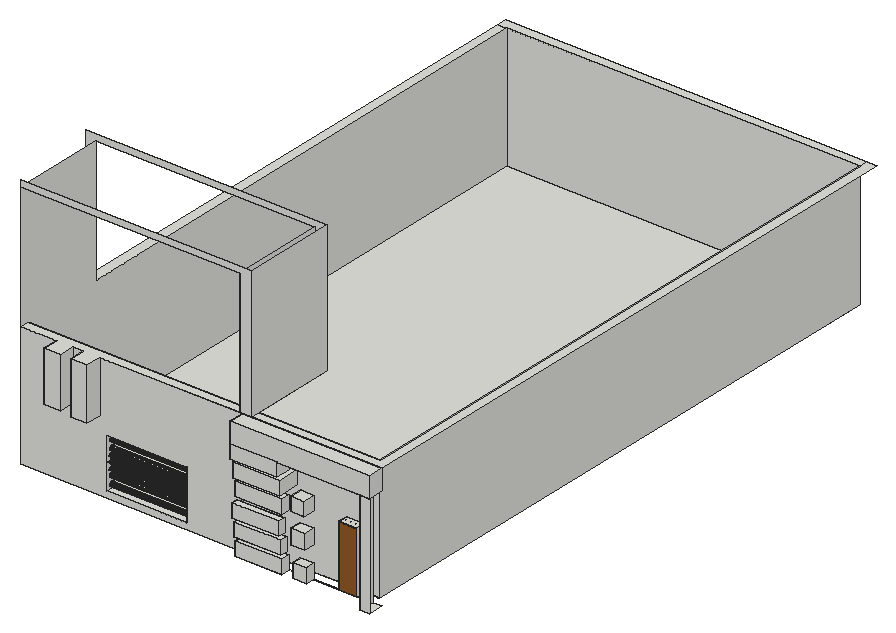
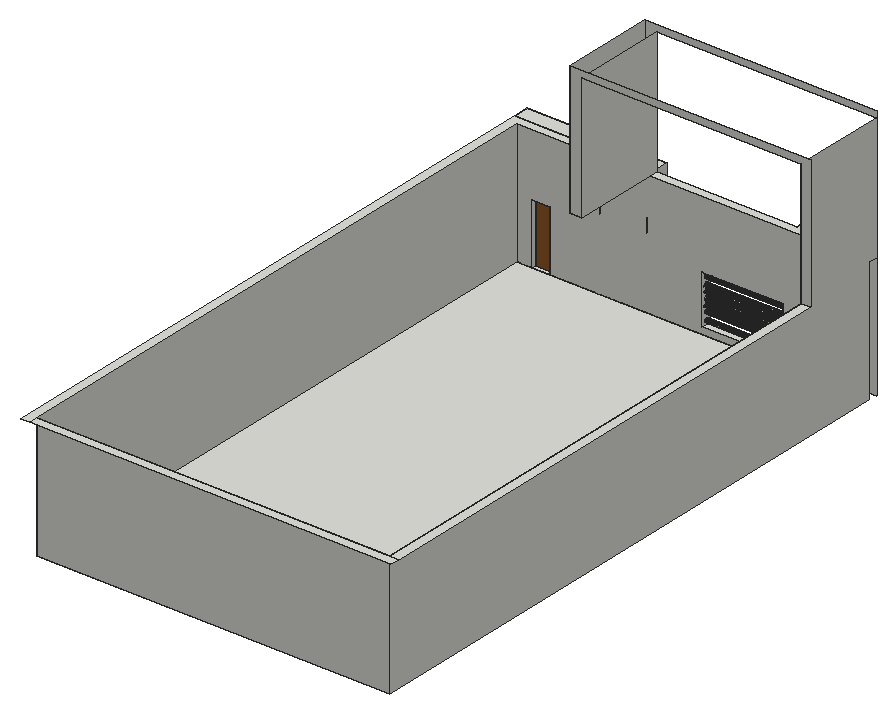
# SketchUp Ruby script. Lengths in inches.
U = 1.inch
M = Sketchup.active_model
def pt(a) = Geom::Point3d.new(a.map { |v| v * U })
def face(e, loops, mat)
  f = e.add_face(loops[0].map { |a| pt(a) })
  loops[1..].each { |l| e.add_face(l.map { |a| pt(a) }).erase! }
  f.material = f.back_material = mat if mat
  f
end
# faces: each face lists its corners as indices into pts; further lists are holes
def faces(e, pts, list, mat = nil) = list.each { |f| face(e, (f[0].is_a?(Array) ? f : [f]).map { |l| l.map { |i| pts[i] } }, mat) }
# xy, xz, yz: faces in a plane at the given z, y or x. An outline is a flat list of corners, or four numbers for a rectangle; further outlines are holes
def ring(l) = l.size == 4 ? [[l[0], l[1]], [l[2], l[1]], [l[2], l[3]], [l[0], l[3]]] : l.each_slice(2).to_a
def flat(e, list, mat, &to3) = list.each { |f| face(e, (f[0].is_a?(Array) ? f : [f]).map { |l| ring(l).map { |u, v| to3.(u, v) } }, mat) }
def xy(e, z, list, mat = nil) = flat(e, list, mat) { |x, y| [x, y, z] }
def xz(e, y, list, mat = nil) = flat(e, list, mat) { |x, z| [x, y, z] }
def yz(e, x, list, mat = nil) = flat(e, list, mat) { |y, z| [x, y, z] }
def lines(e, pts, list) = list.each { |a, b| e.add_line(pt(pts[a]), pt(pts[b])) }
# prism: a flat outline (further loops are holes) pulled along v
def prism(e, loops, v, mat = nil)
  f = face(e, loops, mat); d = Geom::Vector3d.new(v.map { |x| x * U })
  f.pushpull(f.normal.samedirection?(d) ? d.length : -d.length)
end
def box(e, o, s, mat = nil) = prism(e, [[o, [o[0] + s[0], o[1], o[2]], [o[0] + s[0], o[1] + s[1], o[2]], [o[0], o[1] + s[1], o[2]]]], [0, 0, s[2]], mat)
def at(x, y, z, deg = 0) = Geom::Transformation.translation(pt([x, y, z])) * Geom::Transformation.rotation(ORIGIN, Z_AXIS, deg.degrees)
def axes(o, x, y, z) = Geom::Transformation.new([*x, 0, *y, 0, *z, 0, *pt(o).to_a, 1])
def part(name) = M.definitions.add(name)
# library, detail: a bought-in or finely detailed component or shape, given as its bounding box
def library(name, o, s) = part(name).tap { |d| box(d.entities, o, s) }
def detail(e, o, s) = box(e.add_group.entities, o, s)
def put(e, d, t, mat = nil) = e.add_instance(d, t).tap { |i| i.material = mat if mat }
def group(e, t, mat = nil) = e.add_group.tap { |g| g.transformation = t; g.material = mat if mat }.entities
root = M.entities
M.materials.add("[Wood Floor Parquet]").color = [145, 89, 39]
c1 = part("ZZZ")
g1 = group(c1.entities,at(61.03,0,0))
box(g1,[-61.03,0,0],[61.03,1.5625,79.28])
box(root,[224.5625,43.74,143.55],[45.75,6.75,13.12])
box(root,[224.5625,41.22,160.97],[45.75,6.32,13.13])
xy(root,126,[[9.02,62.875,351,644.4375]])
xy(root,126.125,[[351,38.75,360,53.4375],[224.5625,44.875,224.5625,53.875,318.32,53.875,318.32,53.4375,270.3125,53.4375,270.3125,44.875],[335.64,53.4375,351,53.875],[318.32,53.875,335.64,62.875]])
xy(root,127.16,[[281.07,44.125,294.45,53.4375]])
xy(root,132.42,[[92.77,53.875,170.95,62.875]])
xy(root,139.25,[[224.5625,44.875,270.3125,53.4375]])
xy(root,140.53,[[281.07,44.125,294.45,53.4375]])
xy(root,156.97,[[280.4375,42.25,294.5,53.4375]])
xy(root,171.03,[[280.4375,42.25,294.5,53.4375]])
xy(root,178.4,[[224.5625,44.59,270.3125,53.4375]])
xy(root,180.73,[[92.77,53.875,170.95,62.875]])
xy(root,185.5,[[318.32,53.4375,335.64,62.875]])
xy(root,186.3,[[281.15,41.8125,294.21,53.4375]])
xy(root,191.52,[[224.5625,44.59,270.3125,53.4375]])
xy(root,195.5625,[[70.08,38.75,85.7,53.875]])
xy(root,195.82,[[224.5625,41.64,270.3125,62.57]])
xy(root,197.1875,[[43.99,38.75,60.12,53.875]])
xy(root,199.36,[[281.15,41.8125,294.21,53.4375]])
xy(root,208.95,[[224.5625,41.64,270.3125,62.57]])
xy(root,213.25,[[224.5625,38.6875,270.3125,53.4375]])
xy(root,226.37,[[224.5625,38.6875,270.3125,53.4375],[270.3125,38.6875,270.3125,53.4375,351,53.4375,351,38.75,360,38.75,360,38.6875],[351,38.75,360,53.4375]])
xy(root,246,[[224.5625,38.6875,360,53.875],[43.99,38.75,60.12,38.75,60.12,53.875,70.08,53.875,70.08,38.75,85.7,38.75,85.7,53.875,221.54,53.875,221.54,62.875,9.02,62.875,9.02,53.875,43.99,53.875],[221.54,53.875,233.71,62.875],[233.71,53.875,360,53.875,360,653.4375,351,653.4375,351,62.875,233.71,62.875],[221.54,62.875,233.71,144.86],
  [0,144.86,9.02,644.4375],[0,644.4375,351,653.4375]])
xz(root,38.6875,[[224.5625,213.25,270.3125,226.37],[224.5625,226.37,360,246]])
xz(root,38.75,[[351,126.125,360,226.37],[70.08,195.5625,85.7,246],[43.99,197.1875,60.12,246]])
xz(root,41.64,[[224.5625,195.82,270.3125,208.95]])
xz(root,41.8125,[[281.15,186.3,294.21,199.36]])
xz(root,42.25,[[280.4375,156.97,294.5,171.03]])
xz(root,44.125,[[281.07,127.16,294.45,140.53]])
xz(root,44.59,[[224.5625,178.4,270.3125,191.52]])
xz(root,44.875,[[224.5625,126.125,270.3125,139.25]])
xz(root,53.875,[[[9.02,126.125,224.5625,126.125,224.5625,246,85.7,246,85.7,195.5625,70.08,195.5625,70.08,246,60.12,246,60.12,197.1875,43.99,197.1875,43.99,246,9.02,246],[92.77,132.42,170.95,180.73]],[221.54,246,233.71,246,233.71,373.61,9.02,373.61,9.02,367.15,221.54,367.15]])
xz(root,62.57,[[224.5625,195.82,270.3125,208.95]])
xz(root,62.875,[[9.02,126,351,126.125],[[9.02,126.125,9.02,246,351,246,351,126.125,335.64,126.125,335.64,185.5,318.32,185.5,318.32,126.125],[92.77,132.42,170.95,180.73]]])
xz(root,144.86,[[0,246,0,373.61,233.71,373.61,233.71,246,221.54,246,221.54,367.15,9.02,367.15,9.02,246]])
xz(root,644.4375,[[9.02,126,351,246]])
yz(root,9.02,[[62.875,126,644.4375,126,644.4375,246,144.86,246,144.86,367.15,53.875,367.15,53.875,246,62.875,246]])
yz(root,43.99,[[38.75,197.1875,53.875,246]])
yz(root,60.12,[[38.75,197.1875,53.875,246]])
yz(root,70.08,[[38.75,195.5625,53.875,246]])
yz(root,85.7,[[38.75,195.5625,53.875,246]])
yz(root,92.77,[[53.875,132.42,62.875,180.73]])
yz(root,170.95,[[53.875,132.42,62.875,180.73]])
yz(root,221.54,[[53.875,246,144.86,367.15]])
yz(root,224.5625,[[44.875,126.125,44.875,139.25,53.4375,139.25,53.4375,195.82,53.875,195.82,53.875,126.125],[44.59,178.4,53.4375,191.52],[41.64,195.82,53.4375,208.95],[53.4375,195.82,53.875,208.95],[53.875,195.82,62.57,208.95],
  [53.4375,208.95,53.4375,213.25,38.6875,213.25,38.6875,246,53.875,246,53.875,208.95]])
yz(root,233.71,[[53.875,246,144.86,373.61]])
yz(root,270.3125,[[44.875,126.125,53.4375,139.25],[44.59,178.4,53.4375,191.52],[41.64,195.82,62.57,208.95],[38.6875,213.25,53.4375,226.37]])
yz(root,280.4375,[[42.25,156.97,53.4375,171.03]])
yz(root,281.07,[[44.125,127.16,53.4375,140.53]])
yz(root,281.15,[[41.8125,186.3,53.4375,199.36]])
yz(root,294.21,[[41.8125,186.3,53.4375,199.36]])
yz(root,294.45,[[44.125,127.16,53.4375,140.53]])
yz(root,294.5,[[42.25,156.97,53.4375,171.03]])
yz(root,318.32,[[53.4375,126.125,62.875,185.5]])
yz(root,335.64,[[53.4375,126.125,62.875,185.5]])
yz(root,351,[[62.875,126,644.4375,246],[38.75,126.125,53.4375,226.37]])
yz(root,360,[[38.6875,226.37,53.4375,226.37,53.875,246,38.6875,246]])
p = [[92.77,57.95,135.08],[92.77,58.46,134.97],[171.52,58.46,134.97],[171.52,57.95,135.08],[92.77,58.98,135],[171.52,58.98,135],
  [92.77,59.48,135.16],[171.52,59.48,135.16],[92.77,57.48,135.3125],[171.52,57.48,135.3125],[92.77,59.91,135.45],[171.52,59.91,135.45],
  [92.77,57.09,135.66],[171.52,57.09,135.66],[92.77,60.26,135.84],[171.52,60.26,135.84],[92.77,56.81,136.1],[171.52,56.81,136.1],
  [92.77,60.5,136.3],[171.52,60.5,136.3],[92.77,56.65,136.59],[171.52,56.65,136.59],[92.77,60.61,136.8125],[171.52,60.61,136.8125],
  [92.77,56.62,137.11],[171.52,56.62,137.11],[92.77,60.58,137.33],[171.52,60.58,137.33],[92.77,56.72,137.625],[171.52,56.72,137.625],
  [92.77,60.41,137.83],[171.52,60.41,137.83],[92.77,56.96,138.09],[171.52,56.96,138.09],[92.77,60.13,138.27],[171.52,60.13,138.27],
  [92.77,57.31,138.48],[171.52,57.31,138.48],[92.77,59.74,138.61],[171.52,59.74,138.61],[92.77,57.74,138.77],[171.52,57.74,138.77],
  [92.77,59.27,138.85],[171.52,59.27,138.85],[92.77,58.24,138.93],[171.52,58.24,138.93],[92.77,58.76,138.96],[171.52,58.76,138.96],
  [92.77,57.79,142.92],[92.77,58.3,142.82],[171.52,58.3,142.82],[171.52,57.79,142.92],[92.77,58.82,142.85],[171.52,58.82,142.85],
  [92.77,59.31,143.01],[171.52,59.31,143.01],[92.77,57.32,143.16],[171.52,57.32,143.16],[92.77,59.75,143.3],[171.52,59.75,143.3],
  [92.77,56.93,143.51],[171.52,56.93,143.51],[92.77,60.1,143.68],[171.52,60.1,143.68],[92.77,56.65,143.95],[171.52,56.65,143.95],
  [92.77,60.34,144.15],[171.52,60.34,144.15],[92.77,56.48,144.44],[171.52,56.48,144.44],[92.77,60.44,144.66],[171.52,60.44,144.66],
  [92.77,56.45,144.96],[171.52,56.45,144.96],[92.77,60.41,145.18],[171.52,60.41,145.18],[92.77,56.5625,145.47],[171.52,56.5625,145.47],
  [92.77,60.25,145.68],[171.52,60.25,145.68],[92.77,56.8,145.94],[171.52,56.8,145.94],[92.77,59.96,146.12],[171.52,59.96,146.12],
  [92.77,57.14,146.33],[171.52,57.14,146.33],[92.77,59.58,146.46],[171.52,59.58,146.46],[92.77,57.58,146.61],[171.52,57.58,146.61],
  [92.77,59.11,146.7],[171.52,59.11,146.7],[92.77,58.08,146.78],[171.52,58.08,146.78],[92.77,58.6,146.81],[171.52,58.6,146.81],
  [92.77,57.95,148.64],[92.77,58.46,148.53],[171.52,58.46,148.53],[171.52,57.95,148.64],[92.77,58.98,148.56],[171.52,58.98,148.56],
  [92.77,57.48,148.875],[171.52,57.48,148.875],[92.77,59.48,148.72],[171.52,59.48,148.72],[92.77,59.91,149.01],[171.52,59.91,149.01],
  [92.77,57.09,149.22],[171.52,57.09,149.22],[92.77,60.26,149.4],[171.52,60.26,149.4],[92.77,56.81,149.66],[171.52,56.81,149.66],
  [92.77,60.5,149.86],[171.52,60.5,149.86],[92.77,56.65,150.15],[171.52,56.65,150.15],[92.77,60.61,150.375],[171.52,60.61,150.375],
  [92.77,56.62,150.68],[171.52,56.62,150.68],[92.77,60.58,150.9],[171.52,60.58,150.9],[92.77,56.72,151.1875],[171.52,56.72,151.1875],
  [92.77,60.41,151.39],[171.52,60.41,151.39],[92.77,56.96,151.65],[171.52,56.96,151.65],[92.77,60.13,151.83],[171.52,60.13,151.83],
  [92.77,57.31,152.04],[171.52,57.31,152.04],[92.77,59.74,152.18],[171.52,59.74,152.18],[92.77,57.74,152.33],[171.52,57.74,152.33],
  [92.77,59.27,152.41],[171.52,59.27,152.41],[92.77,58.24,152.49],[171.52,58.24,152.49],[92.77,58.76,152.52],[171.52,58.76,152.52],
  [91.06,58.11,154.6],[91.06,58.625,154.5],[169.81,58.625,154.5],[169.81,58.11,154.6],[91.06,59.15,154.53],[169.81,59.15,154.53],
  [91.06,59.64,154.69],[169.81,59.64,154.69],[91.06,57.65,154.84],[169.81,57.65,154.84],[91.06,60.08,154.98],[169.81,60.08,154.98],
  [91.06,57.26,155.1875],[169.81,57.26,155.1875],[91.06,60.43,155.36],[169.81,60.43,155.36],[91.06,56.97,155.625],[169.81,56.97,155.625],
  [91.06,60.66,155.83],[169.81,60.66,155.83],[91.06,56.81,156.12],[169.81,56.81,156.12],[91.06,60.77,156.34],[169.81,60.77,156.34],
  [91.06,56.78,156.64],[169.81,56.78,156.64],[91.06,60.74,156.86],[169.81,60.74,156.86],[91.06,56.89,157.15],[169.81,56.89,157.15],
  [91.06,60.58,157.36],[169.81,60.58,157.36],[91.06,57.125,157.62],[169.81,57.125,157.62],[91.06,60.29,157.8],[169.81,60.29,157.8],
  [91.06,57.47,158.01],[169.81,57.47,158.01],[91.06,59.9,158.14],[169.81,59.9,158.14],[91.06,57.91,158.29],[169.81,57.91,158.29],
  [91.06,59.4375,158.38],[169.81,59.4375,158.38],[91.06,58.4,158.46],[169.81,58.4,158.46],[91.06,58.93,158.49],[169.81,58.93,158.49],
  [92.77,57.95,160.7],[92.77,58.46,160.59],[171.52,58.46,160.59],[171.52,57.95,160.7],[92.77,58.98,160.62],[171.52,58.98,160.62],
  [92.77,59.48,160.79],[171.52,59.48,160.79],[92.77,57.48,160.9375],[171.52,57.48,160.9375],[92.77,59.91,161.07],[171.52,59.91,161.07],
  [92.77,57.09,161.28],[171.52,57.09,161.28],[92.77,60.26,161.46],[171.52,60.26,161.46],[92.77,56.81,161.72],[171.52,56.81,161.72],
  [92.77,60.5,161.93],[171.52,60.5,161.93],[92.77,56.65,162.22],[171.52,56.65,162.22],[92.77,60.61,162.4375],[171.52,60.61,162.4375],
  [92.77,56.62,162.74],[171.52,56.62,162.74],[92.77,60.58,162.96],[171.52,60.58,162.96],[92.77,56.72,163.25],[171.52,56.72,163.25],
  [92.77,60.41,163.45],[171.52,60.41,163.45],[92.77,56.96,163.72],[171.52,56.96,163.72],[92.77,60.13,163.89],[171.52,60.13,163.89],
  [92.77,57.31,164.1],[171.52,57.31,164.1],[92.77,59.74,164.24],[171.52,59.74,164.24],[92.77,57.74,164.39],[171.52,57.74,164.39],
  [92.77,59.27,164.48],[171.52,59.27,164.48],[92.77,58.24,164.55],[171.52,58.24,164.55],[92.77,58.76,164.58],[171.52,58.76,164.58],
  [92.77,57.95,166.14],[92.77,58.46,166.03],[171.52,58.46,166.03],[171.52,57.95,166.14],[92.77,58.98,166.06],[171.52,58.98,166.06],
  [92.77,57.48,166.375],[171.52,57.48,166.375],[92.77,59.48,166.22],[171.52,59.48,166.22],[92.77,59.91,166.51],[171.52,59.91,166.51],
  [92.77,57.09,166.72],[171.52,57.09,166.72],[92.77,60.26,166.9],[171.52,60.26,166.9],[92.77,56.81,167.16],[171.52,56.81,167.16],
  [92.77,60.5,167.36],[171.52,60.5,167.36],[92.77,56.65,167.65],[171.52,56.65,167.65],[92.77,60.61,167.875],[171.52,60.61,167.875],
  [92.77,56.62,168.18],[171.52,56.62,168.18],[92.77,60.58,168.4],[171.52,60.58,168.4],[92.77,56.72,168.6875],[171.52,56.72,168.6875],
  [92.77,60.41,168.89],[171.52,60.41,168.89],[92.77,56.96,169.15],[171.52,56.96,169.15],[92.77,60.13,169.33],[171.52,60.13,169.33],
  [92.77,57.31,169.54],[171.52,57.31,169.54],[92.77,59.74,169.68],[171.52,59.74,169.68],[92.77,57.74,169.83],[171.52,57.74,169.83],
  [92.77,59.27,169.91],[171.52,59.27,169.91],[92.77,58.24,169.99],[171.52,58.24,169.99],[92.77,58.76,170.02],[171.52,58.76,170.02],
  [92.33,58.14,173.93],[92.33,58.65,173.82],[171.08,58.65,173.82],[171.08,58.14,173.93],[92.33,59.17,173.85],[171.08,59.17,173.85],
  [92.33,59.67,174.01],[171.08,59.67,174.01],[92.33,57.67,174.16],[171.08,57.67,174.16],[92.33,60.1,174.3],[171.08,60.1,174.3],
  [92.33,57.28,174.51],[171.08,57.28,174.51],[92.33,60.45,174.6875],[171.08,60.45,174.6875],[92.33,57,174.95],[171.08,57,174.95],
  [92.33,60.6875,175.15],[171.08,60.6875,175.15],[92.33,56.83,175.44],[171.08,56.83,175.44],[92.33,60.79,175.66],[171.08,60.79,175.66],
  [92.33,56.8,175.97],[171.08,56.8,175.97],[92.33,60.76,176.19],[171.08,60.76,176.19],[92.33,56.91,176.48],[171.08,56.91,176.48],
  [92.33,60.6,176.68],[171.08,60.6,176.68],[92.33,57.15,176.94],[171.08,57.15,176.94],[92.33,60.32,177.12],[171.08,60.32,177.12],
  [92.33,57.5,177.33],[171.08,57.5,177.33],[92.33,59.93,177.47],[171.08,59.93,177.47],[92.33,57.93,177.62],[171.08,57.93,177.62],
  [92.33,59.46,177.7],[171.08,59.46,177.7],[92.33,58.43,177.78],[171.08,58.43,177.78],[92.33,58.95,177.81],[171.08,58.95,177.81],
  [360,53.4375,226.37],[360,53.875,246],[233.71,53.875,246],[224.5625,53.875,246],[224.34,53.875,246],[224.34,53.4375,226.37],
  [224.5625,53.4375,226.37],[270.3125,53.4375,226.37],[351,53.4375,226.37]]
faces(root,p,[[0,1,2,3],[1,4,5,2],[4,6,7,5],[8,0,3,9],[6,10,11,7],[12,8,9,13],[10,14,15,11],[16,12,13,17],
  [14,18,19,15],[20,16,17,21],[18,22,23,19],[24,20,21,25],[22,26,27,23],[28,24,25,29],[26,30,31,27],[32,28,29,33],
  [30,34,35,31],[36,32,33,37],[34,38,39,35],[40,36,37,41],[38,42,43,39],[44,40,41,45],[46,44,45,47],[42,46,47,43],
  [48,49,50,51],[49,52,53,50],[52,54,55,53],[56,48,51,57],[54,58,59,55],[60,56,57,61],[58,62,63,59],[64,60,61,65],
  [62,66,67,63],[68,64,65,69],[66,70,71,67],[72,68,69,73],[70,74,75,71],[76,72,73,77],[74,78,79,75],[80,76,77,81],
  [78,82,83,79],[84,80,81,85],[82,86,87,83],[88,84,85,89],[86,90,91,87],[92,88,89,93],[90,94,95,91],[94,92,93,95],
  [96,97,98,99],[97,100,101,98],[102,96,99,103],[100,104,105,101],[104,106,107,105],[108,102,103,109],[106,110,111,107],[112,108,109,113],
  [110,114,115,111],[116,112,113,117],[114,118,119,115],[120,116,117,121],[118,122,123,119],[124,120,121,125],[122,126,127,123],[128,124,125,129],
  [126,130,131,127],[132,128,129,133],[130,134,135,131],[136,132,133,137],[134,138,139,135],[140,136,137,141],[138,142,143,139],[142,140,141,143],
  [144,145,146,147],[145,148,149,146],[148,150,151,149],[152,144,147,153],[150,154,155,151],[156,152,153,157],[154,158,159,155],[160,156,157,161],
  [158,162,163,159],[164,160,161,165],[162,166,167,163],[168,164,165,169],[166,170,171,167],[172,168,169,173],[170,174,175,171],[176,172,173,177],
  [174,178,179,175],[180,176,177,181],[178,182,183,179],[184,180,181,185],[182,186,187,183],[188,184,185,189],[186,190,191,187],[190,188,189,191],
  [192,193,194,195],[193,196,197,194],[196,198,199,197],[200,192,195,201],[198,202,203,199],[204,200,201,205],[202,206,207,203],[208,204,205,209],
  [206,210,211,207],[212,208,209,213],[210,214,215,211],[216,212,213,217],[214,218,219,215],[220,216,217,221],[218,222,223,219],[224,220,221,225],
  [222,226,227,223],[228,224,225,229],[226,230,231,227],[232,228,229,233],[230,234,235,231],[236,232,233,237],[234,238,239,235],[238,236,237,239],
  [240,241,242,243],[241,244,245,242],[246,240,243,247],[244,248,249,245],[248,250,251,249],[252,246,247,253],[250,254,255,251],[256,252,253,257],
  [254,258,259,255],[260,256,257,261],[258,262,263,259],[264,260,261,265],[262,266,267,263],[268,264,265,269],[266,270,271,267],[272,268,269,273],
  [270,274,275,271],[276,272,273,277],[274,278,279,275],[280,276,277,281],[278,282,283,279],[284,280,281,285],[282,286,287,283],[286,284,285,287],
  [288,289,290,291],[289,292,293,290],[292,294,295,293],[296,288,291,297],[294,298,299,295],[300,296,297,301],[298,302,303,299],[304,300,301,305],
  [302,306,307,303],[308,304,305,309],[306,310,311,307],[312,308,309,313],[310,314,315,311],[316,312,313,317],[314,318,319,315],[320,316,317,321],
  [318,322,323,319],[324,320,321,325],[322,326,327,323],[328,324,325,329],[326,330,331,327],[332,328,329,333],[330,334,335,331],[334,332,333,335],
  [336,337,338,339,340,341,342,343,344]])
put(root,c1,axes([318.33,53.54,126.15],[0.28354,0,0],[0,3.23919,0],[0,0,0.74546]),"[Wood Floor Parquet]")
